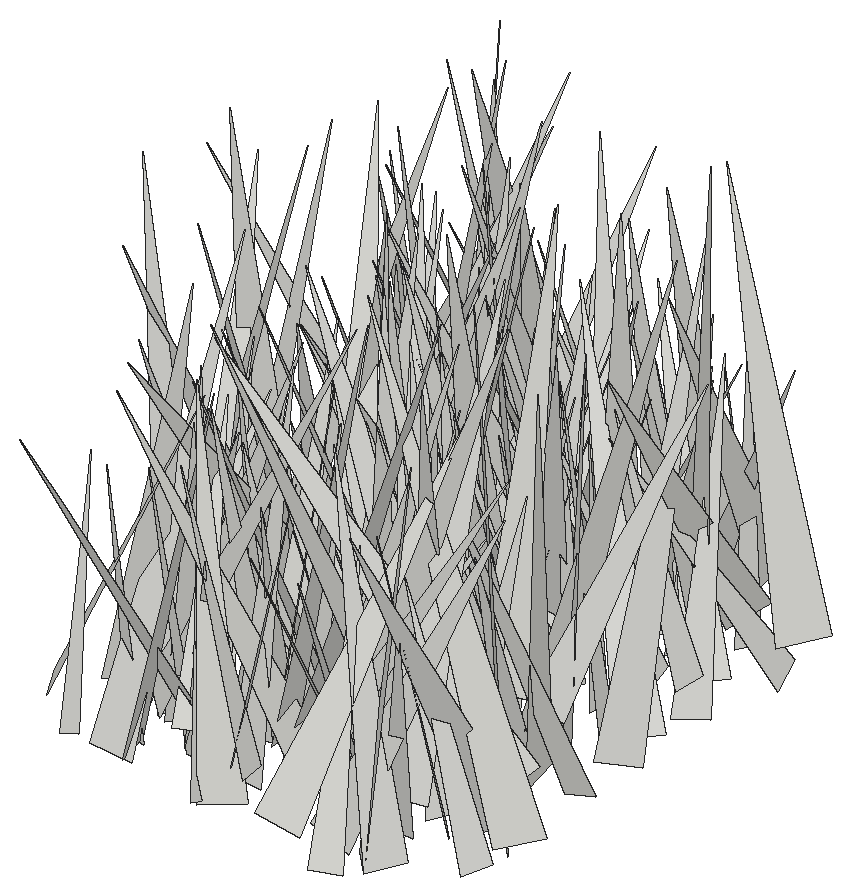
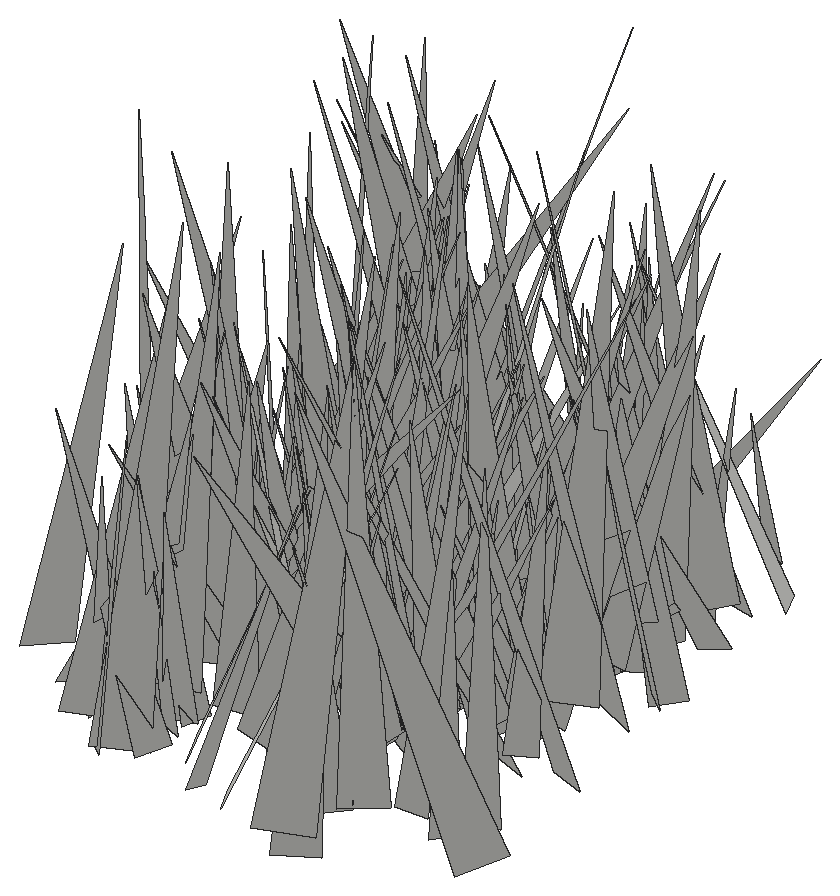
# SketchUp Ruby script. Lengths in inches.
U = 1.inch
M = Sketchup.active_model
def pt(a) = Geom::Point3d.new(a.map { |v| v * U })
def face(e, loops, mat)
  f = e.add_face(loops[0].map { |a| pt(a) })
  loops[1..].each { |l| e.add_face(l.map { |a| pt(a) }).erase! }
  f.material = f.back_material = mat if mat
  f
end
# faces: each face lists its corners as indices into pts; further lists are holes
def faces(e, pts, list, mat = nil) = list.each { |f| face(e, (f[0].is_a?(Array) ? f : [f]).map { |l| l.map { |i| pts[i] } }, mat) }
# xy, xz, yz: faces in a plane at the given z, y or x. An outline is a flat list of corners, or four numbers for a rectangle; further outlines are holes
def ring(l) = l.size == 4 ? [[l[0], l[1]], [l[2], l[1]], [l[2], l[3]], [l[0], l[3]]] : l.each_slice(2).to_a
def flat(e, list, mat, &to3) = list.each { |f| face(e, (f[0].is_a?(Array) ? f : [f]).map { |l| ring(l).map { |u, v| to3.(u, v) } }, mat) }
def xy(e, z, list, mat = nil) = flat(e, list, mat) { |x, y| [x, y, z] }
def xz(e, y, list, mat = nil) = flat(e, list, mat) { |x, z| [x, y, z] }
def yz(e, x, list, mat = nil) = flat(e, list, mat) { |y, z| [x, y, z] }
def lines(e, pts, list) = list.each { |a, b| e.add_line(pt(pts[a]), pt(pts[b])) }
# prism: a flat outline (further loops are holes) pulled along v
def prism(e, loops, v, mat = nil)
  f = face(e, loops, mat); d = Geom::Vector3d.new(v.map { |x| x * U })
  f.pushpull(f.normal.samedirection?(d) ? d.length : -d.length)
end
def box(e, o, s, mat = nil) = prism(e, [[o, [o[0] + s[0], o[1], o[2]], [o[0] + s[0], o[1] + s[1], o[2]], [o[0], o[1] + s[1], o[2]]]], [0, 0, s[2]], mat)
def at(x, y, z, deg = 0) = Geom::Transformation.translation(pt([x, y, z])) * Geom::Transformation.rotation(ORIGIN, Z_AXIS, deg.degrees)
def axes(o, x, y, z) = Geom::Transformation.new([*x, 0, *y, 0, *z, 0, *pt(o).to_a, 1])
def part(name) = M.definitions.add(name)
# library, detail: a bought-in or finely detailed component or shape, given as its bounding box
def library(name, o, s) = part(name).tap { |d| box(d.entities, o, s) }
def detail(e, o, s) = box(e.add_group.entities, o, s)
def put(e, d, t, mat = nil) = e.add_instance(d, t).tap { |i| i.material = mat if mat }
def group(e, t, mat = nil) = e.add_group.tap { |g| g.transformation = t; g.material = mat if mat }.entities
root = M.entities
c1 = part("fur_instance\#9")
p = [[0.8125,0,1.79],[0.67,-0.02,1.48],[0,-0.11,0],[0,0.11,0]]
faces(c1.entities,p,[[0,1,2,3]])
put(root,c1,axes([122.5,103.28,-28.22],[2.81621,-4.35059,0.38195],[-4.36621,-2.81499,0.12899],[-0.09891,0.39082,5.18093]))
put(root,c1,axes([125.08,92.21,-28.22],[-7.4138,3.10521,1.79195],[3.13289,7.61249,-0.22981],[1.74312,-0.47482,8.03455]))
put(root,c1,axes([122.99,104.25,-28.22],[4.3252,-1.84495,1.08949],[-1.74272,-4.45705,-0.62914],[-1.2465,-0.1704,4.65998]))
put(root,c1,axes([124.71,87.48,-27.1],[0.6459,3.9486,0.07217],[3.68247,-0.62859,1.43463],[-1.42692,0.16515,3.73504]))
put(root,c1,axes([122.98,100.89,-27.1],[2.32528,-3.90872,0.2043],[-3.90658,-2.33236,-0.15975],[-0.24182,0.09371,4.54527]))
put(root,c1,axes([123.83,97.73,-27.1],[3.74176,-6.61768,2.63887],[-6.89022,-4.11933,-0.5604],[-1.81167,1.99888,7.58159]))
put(root,c1,axes([124.63,93.51,-28.22],[-3.64093,6.72533,0.73654],[6.73348,3.68347,-0.34805],[0.65778,-0.48058,7.63972]))
put(root,c1,axes([124.44,95.17,-27.1],[0.3349,-5.08877,0.86463],[-5.08924,-0.4702,-0.79617],[-0.86188,0.79915,5.03725]))
put(root,c1,axes([123.36,105.31,-27.1],[-0.67207,-6.04885,0.74296],[-6.03248,0.76649,0.78356],[0.86591,0.6451,6.03542]))
put(root,c1,axes([125.18,97.24,-28.22],[0.28426,-7.43419,0.75555],[-7.30944,-0.43371,-1.51752],[-1.55247,0.68085,7.28321]))
put(root,c1,axes([123.59,95.97,-28.22],[2.95959,7.19025,1.54721],[7.29869,-3.07695,0.338],[-0.90704,-1.29822,7.76818]))
put(root,c1,axes([121.16,104.88,-28.22],[5.54301,-4.89223,1.08245],[-4.92161,-5.01325,2.54471],[0.93987,2.60075,6.94141]))
put(root,c1,axes([121.99,96.09,-27.1],[6.05057,5.41917,1.99571],[5.77348,-5.74186,-1.9125],[-0.1309,-2.76104,7.89425]))
put(root,c1,axes([122.3,99.67,-28.22],[4.03025,7.20792,1.49357],[7.34455,-3.82368,-1.36555],[0.49235,-1.96292,8.14446]))
put(root,c1,axes([126.06,100.875,-27.1],[-4.18794,0.93567,0.33129],[0.9893,4.05153,1.06324],[0.08071,-1.11073,4.15738]))
put(root,c1,axes([125.14,89.89,-28.22],[-1.82115,-3.36265,1.61921],[-3.73204,1.65736,-0.7556],[0.03439,1.7865,3.74875]))
put(root,c1,axes([127.07,101.125,-27.1],[-7.35388,-1.92649,0.06127],[-1.88282,7.23164,1.39751],[0.41243,-1.33667,7.47248]))
put(root,c1,axes([124.92,93.42,-28.22],[-4.28711,2.60894,1.39768],[2.40918,4.50508,-1.01958],[1.71929,0.19268,4.91389]))
put(root,c1,axes([122.51,89.43,-27.1],[4.96423,2.67259,0.04648],[2.6631,-4.93667,-0.5706],[0.22978,-0.52435,5.60898]))
put(root,c1,axes([123.82,91.16,-28.22],[-0.74484,5.04348,0.31723],[4.84937,0.80355,-1.38926],[1.42161,-0.09859,4.90524]))
put(root,c1,axes([127.97,90.31,-28.22],[-2.43401,-4.94438,0.27236],[-4.40728,2.02468,-2.63096],[-2.25763,1.37813,4.84245]))
put(root,c1,axes([122.875,94.39,-28.22],[2.55159,-4.81811,0.15811],[-4.66384,-2.42197,1.46026],[1.21971,0.81832,5.25284]))
put(root,c1,axes([125.04,88.91,-28.22],[1.15921,7.66569,0.40932],[7.66684,-1.17697,0.3294],[-0.3873,-0.35503,7.74584]))
put(root,c1,axes([124.57,105.9375,-27.1],[4.01557,-5.25956,2.05629],[-5.53772,-4.16187,0.169],[-1.10676,1.74125,6.61508]))
put(root,c1,axes([124.03,90.97,-27.1],[5.12868,-4.19399,1.94705],[-4.5125,-5.17419,0.74098],[-1.00889,1.82269,6.58361]))
put(root,c1,axes([124.64,99.09,-27.1],[3.47774,-1.50181,0.39234],[-1.2719,-3.30895,-1.39185],[-0.88975,-1.13996,3.5232]))
put(root,c1,axes([124.42,98.15,-28.22],[3.9235,0.14114,0.37721],[0.06723,-3.8717,0.74932],[-0.3971,0.73898,3.85386]))
put(root,c1,axes([127.51,95.6,-28.22],[-3.53449,-6.31522,1.62159],[-6.50822,3.306,-1.31053],[-0.39309,2.04757,7.11738]))
put(root,c1,axes([124.58,102.7,-28.22],[4.94057,6.27292,2.28459],[6.62263,-4.9638,-0.69253],[-0.84236,-2.23369,7.95482]))
put(root,c1,axes([126.96,101.19,-28.22],[-2.82637,-5.01502,0.69558],[-5.06125,2.81969,-0.23605],[0.13409,0.7222,5.75179]))
put(root,c1,axes([124.77,105.6875,-27.1],[4.05285,-0.43746,0.41546],[-0.3233,-3.95717,-1.01285],[-0.50937,-0.96903,3.94856]))
put(root,c1,axes([124.27,99.93,-28.22],[3.274,7.7332,0.0389],[7.72076,-3.26624,-0.49451],[0.44025,-0.22856,8.38313]))
put(root,c1,axes([126.52,100.1875,-27.1],[-2.91757,4.706,0.99504],[4.75363,2.9987,-0.24403],[0.73452,-0.71423,5.53165]))
put(root,c1,axes([127.03,90.125,-28.22],[-1.86227,-3.58892,1.59018],[-3.91628,1.57852,-1.02377],[-0.26793,1.87217,3.91156]))
put(root,c1,axes([124.77,92.31,-27.1],[4.76351,-2.22786,1.63166],[-2.67424,-4.53288,1.61806],[-0.68857,2.19233,5.00362]))
put(root,c1,axes([125.45,98.64,-28.22],[6.28963,-0.96384,2.1084],[-1.07131,-6.61487,0.17192],[-2.05588,0.49827,6.36073]))
put(root,c1,axes([126.16,97.22,-27.1],[6.60243,-3.6292,1.16999],[-2.40466,-5.77841,-4.35427],[-2.95933,-3.40161,6.14845]))
put(root,c1,axes([127.39,96.2,-28.22],[-5.56313,6.05819,1.00831],[6.02083,5.64819,-0.71719],[1.2116,-0.25113,8.19364]))
put(root,c1,axes([125.4375,108.43,-27.1],[4.78768,-6.87101,0.53821],[-6.76798,-4.81092,-1.21319],[-1.30189,-0.25808,8.28619]))
put(root,c1,axes([127.04,93.37,-28.22],[-5.00491,-0.78513,1.46412],[-0.94309,5.16869,-0.45214],[1.36772,0.69095,5.0459]))
put(root,c1,axes([127.14,102.01,-27.1],[5.31118,5.11176,2.74997],[4.78098,-5.96627,1.85658],[-3.29161,-0.41778,7.13385]))
put(root,c1,axes([125.53,91.66,-28.22],[4.04014,-3.74392,1.13553],[-3.80741,-4.13804,-0.09691],[-0.90002,0.69913,5.50729]))
put(root,c1,axes([128.55,99.65,-28.22],[-7.00273,-0.39667,0.95685],[-0.59042,6.90153,-1.45992],[0.85107,1.52402,6.86034]))
put(root,c1,axes([127.22,98.15,-28.22],[-3.60239,-0.15597,0.87969],[-0.19043,3.7046,-0.12301],[0.87288,0.16452,3.60367]))
put(root,c1,axes([125.39,89.45,-28.22],[5.7925,1.49056,1.34896],[1.52882,-5.93778,-0.00376],[-1.30544,-0.3399,5.9812]))
put(root,c1,axes([127.21,89.71,-27.1],[-2.44616,4.11048,0.29857],[4.09909,2.46258,-0.31948],[0.42742,-0.0923,4.7726]))
put(root,c1,axes([125.58,107.7,-28.22],[4.30968,-5.09044,0.61484],[-5.06109,-4.35201,-0.55619],[-0.82219,0.10671,6.64655]))
put(root,c1,axes([127.07,94.18,-27.1],[1.11597,-3.30458,1.27259],[-3.40234,-1.37051,-0.57526],[-0.98175,0.99326,3.44016]))
put(root,c1,axes([127.21,93.55,-28.22],[-4.48164,3.41054,1.04148],[3.17852,4.57879,-1.31654],[1.61662,0.45221,5.47573]))
put(root,c1,axes([129.2,103.3,-27.1],[-7.32876,-0.97242,0.83606],[-1.07916,7.29688,-0.97277],[0.69283,1.07947,7.32872]))
put(root,c1,axes([125.67,95.92,-28.22],[4.93042,2.67254,1.54888],[2.99605,-4.84755,-1.1728],[-0.75178,-1.79146,5.48417]))
put(root,c1,axes([128.22,104.02,-28.22],[-4.66446,-0.17714,0.77084],[-0.14932,4.72517,0.1823],[0.77671,-0.15541,4.66426]))
put(root,c1,axes([124.67,100.06,-27.1],[6.16079,-1.33707,0.34037],[-1.37023,-6.11166,0.79308],[-0.16154,0.84778,6.25413]))
put(root,c1,axes([127.18,97.35,-27.1],[-2.4025,-2.92839,0.44923],[-2.80853,2.4353,0.85486],[0.94311,-0.20767,3.69008]))
put(root,c1,axes([128.77,88.4,-28.22],[-6.05954,0.33778,0.89505],[0.02694,5.79744,-2.00555],[0.95629,1.97708,5.728]))
put(root,c1,axes([128.68,100.66,-27.1],[0.56796,-5.36738,0.34113],[-5.01782,-0.65229,-1.90884],[-1.93561,0.11605,5.04853]))
put(root,c1,axes([129.16,106.4375,-28.22],[-5.15654,-2.89646,0.02201],[-2.88562,5.14083,0.47427],[0.2514,-0.40276,5.89529]))
put(root,c1,axes([128.62,101.76,-27.1],[1.86893,4.92203,0.04113],[4.36091,-1.67616,2.42774],[-2.28266,0.8277,4.67176]))
put(root,c1,axes([126.3125,105.0625,-28.22],[3.18493,-3.37138,0.77047],[-3.44968,-3.17103,0.3845],[-0.24394,0.82581,4.62191]))
put(root,c1,axes([126.41,102.44,-27.1],[5.41159,0.09186,1.28906],[0.07062,-5.56242,0.09991],[-1.29039,0.08081,5.41145]))
put(root,c1,axes([127.11,102.1,-27.1],[-1.46748,5.77462,2.34569],[6.13429,1.76496,-0.50731],[1.10405,-2.13089,5.93652]))
put(root,c1,axes([127.42,100.625,-27.1],[0.8568,-5.86099,0.80486],[-5.91149,-0.87995,-0.11477],[-0.231,0.77949,5.92218]))
put(root,c1,axes([128.22,105.14,-27.1],[-3.59271,-3.52154,0.36411],[-3.38524,3.56898,1.11534],[1.03633,-0.55007,4.90559]))
put(root,c1,axes([128.3,92.16,-28.22],[0.40641,-5.35004,1.66525],[-5.54368,-0.62666,-0.66032],[-0.81458,1.59547,5.32467]))
put(root,c1,axes([126.89,90.57,-28.22],[2.03296,-3.43324,0.36978],[-3.45285,-2.01606,0.26469],[0.04074,0.45292,3.9812]))
put(root,c1,axes([127.39,91.125,-28.22],[2.94995,3.39967,1.09614],[3.50655,-3.02709,-0.04841],[-0.68072,-0.86052,4.50085]))
put(root,c1,axes([129.93,95.78,-28.22],[-5.4054,2.23783,0.44972],[2.26041,5.40869,0.2551],[0.31726,-0.40826,5.84475]))
put(root,c1,axes([129.29,104.84,-27.1],[-0.74587,-6.40704,1.23448],[-6.45249,0.53969,-1.09751],[-0.96927,1.33753,6.35625]))
put(root,c1,axes([127.55,101,-28.22],[-5.17652,4.83446,1.05401],[3.91261,4.93311,-3.41105],[3.02894,1.88989,6.20751]))
put(root,c1,axes([130.46,92.89,-28.22],[-2.94744,-5.34651,0.76174],[-5.29498,2.69026,-1.60576],[-1.06233,1.42484,5.89017]))
put(root,c1,axes([126.07,99.46,-27.1],[3.27115,-5.93629,2.22387],[-6.24966,-2.60094,2.25],[1.06155,2.98013,6.39355]))
put(root,c1,axes([130.375,91.33,-28.22],[-6.87561,-0.89332,0.66489],[-0.69538,6.69239,1.80069],[0.86979,-1.71115,6.69549]))
put(root,c1,axes([129.24,88.57,-28.22],[-3.57367,4.96866,1.72232],[5.21894,3.60663,0.42422],[0.64547,-1.65218,6.10563]))
put(root,c1,axes([125.23,90.57,-27.1],[5.08074,5.57509,0.64514],[5.46993,-4.72427,-2.25231],[1.25607,-1.97773,7.19879]))
put(root,c1,axes([131.49,93.66,-28.22],[-5.18196,-4.15409,0.26027],[-4.02731,4.89921,-1.98883],[-1.05116,1.70828,6.3367]))
put(root,c1,axes([129.84,98.58,-28.22],[-7.87878,-1.52664,2.20407],[-1.70967,8.13085,-0.47967],[2.06533,0.90687,8.01097]))
put(root,c1,axes([128.19,92.67,-28.22],[4.42301,-0.66017,1.25029],[-0.31732,-4.46498,-1.23502],[-1.37781,-1.09094,4.29808]))
put(root,c1,axes([130.38,97.59,-27.1],[-4.86082,-0.82699,0.28427],[-0.77768,4.82218,0.73078],[0.39992,-0.67448,4.87621]))
put(root,c1,axes([130.04,88.875,-27.1],[-4.57594,-0.69447,0.70937],[-0.73517,4.61906,-0.2203],[0.6671,0.32667,4.62309]))
put(root,c1,axes([130.01,94.16,-27.1],[1.21236,6.8418,0.01969],[6.58716,-1.17263,1.87473],[-1.84929,0.30844,6.6907]))
put(root,c1,axes([128.9375,89.93,-28.22],[1.06492,5.99669,1.55027],[6.17359,-1.15473,0.22589],[-0.50038,-1.48458,6.08632]))
put(root,c1,axes([129.68,96.99,-28.22],[-5.57338,-5.53642,0.81265],[-5.27737,5.58191,1.83481],[1.86058,-0.75178,7.63858]))
put(root,c1,axes([128.1,98.21,-27.1],[7.25129,-2.23194,2.73946],[-2.93898,-7.28136,1.84704],[-1.96177,2.6585,7.35875]))
put(root,c1,axes([134.1875,100.6,-27.1],[-5.38862,-5.55187,0.24968],[-4.68183,4.34761,-4.37054],[-2.99434,3.19341,6.38427]))
put(root,c1,axes([130.23,106.39,-28.22],[-4.47409,-0.55232,0.95951],[-0.288,4.43762,1.21151],[1.069,-1.11608,4.34221]))
put(root,c1,axes([129.16,94.58,-28.22],[5.828,-3.21448,3.45143],[-4.0564,-6.21538,1.06086],[-2.40642,2.69201,6.57061]))
put(root,c1,axes([130.8,94.84,-28.22],[5.10712,-2.96498,5.20518],[-4.57955,-6.3419,0.88079],[-3.86171,3.59957,5.83935]))
put(root,c1,axes([131.67,104.77,-28.22],[-5.05494,-2.22544,0.30278],[-2.23904,4.935,-1.10864],[-0.17591,1.1357,5.41072]))
put(root,c1,axes([131.78,99.42,-27.1],[-4.01783,2.35497,0.3103],[2.27352,3.63609,1.84258],[-0.68795,-1.73727,4.27712]))
put(root,c1,axes([130.64,98.13,-27.1],[-5.01766,-1.40088,1.70753],[-1.93126,4.83928,-1.7049],[1.07162,2.16194,4.92267]))
put(root,c1,axes([129.11,92.55,-27.1],[-3.54773,2.23846,2.32232],[2.39169,4.14191,-0.33862],[2.16418,-0.90784,4.1812]))
put(root,c1,axes([130.97,102,-27.1],[-7.04471,-1.4589,1.32068],[-0.96261,6.83613,2.41686],[1.71638,-2.15394,6.77607]))
put(root,c1,axes([130.78,103.87,-27.1],[-2.14866,5.91991,1.32548],[6.06222,2.04254,0.70466],[-0.22751,-1.48381,6.25824]))
put(root,c1,axes([129.02,101.34,-27.1],[3.30079,2.00098,0.99665],[2.11543,-3.37049,-0.23912],[-0.72261,-0.72685,3.85253]))
put(root,c1,axes([129.34,100.34,-27.1],[2.40943,-6.40182,1.38295],[-6.51779,-2.4885,-0.16399],[-0.64358,1.23501,6.83826]))
put(root,c1,axes([129.16,89.17,-27.1],[-3.23487,-1.73884,2.61208],[-2.22596,3.91581,-0.14997],[2.2117,1.39779,3.66954]))
put(root,c1,axes([132.13,94.79,-27.1],[-5.92654,3.46188,1.28835],[3.68281,5.72588,1.55549],[0.28525,-1.99951,6.68498]))
put(root,c1,axes([130.74,99.92,-27.1],[3.92843,5.06138,3.38638],[5.5366,-4.64662,0.52215],[-2.53598,-2.30413,6.38572]))
put(root,c1,axes([130.04,101.38,-28.22],[-3.2792,-1.26365,1.37089],[-0.97388,3.52607,0.9207],[1.58988,-0.44645,3.3915]))
put(root,c1,axes([133.17,98.52,-28.22],[-4.03956,-5.75099,0.92293],[-5.66396,3.6166,-2.25467],[-1.3584,2.0224,6.65646]))
put(root,c1,axes([129.85,96.04,-27.1],[-4.92901,3.2655,3.81824],[4.17297,5.6397,0.56365],[2.798,-2.65855,5.88565]))
put(root,c1,axes([129.49,91.01,-27.1],[6.35559,1.23086,1.81432],[1.1106,-6.60444,0.5901],[-1.89033,0.25813,6.44673]))
put(root,c1,axes([131.25,99.02,-28.22],[4.80769,-4.80499,2.60276],[-4.52111,-5.44469,-1.70033],[-3.0695,0.49361,6.58109]))
put(root,c1,axes([130.94,99.37,-28.22],[-5.21619,-2.22313,1.39253],[-1.54183,5.10575,2.37575],[2.12232,-1.75473,5.14847]))
put(root,c1,axes([130.77,94.09,-27.1],[4.6761,-4.10232,2.76945],[-4.45315,-5.14998,-0.1096],[-2.16064,1.73593,6.21956]))
put(root,c1,axes([131.96,97.45,-28.22],[0.51601,7.02264,0.2402],[6.84431,-0.55684,1.57697],[-1.5908,-0.11784,6.86272]))
put(root,c1,axes([131.39,99.12,-27.1],[2.56304,5.03632,1.18387],[4.82189,-2.80423,1.49027],[-1.87495,-0.32715,5.45094]))
put(root,c1,axes([132.99,94.48,-28.22],[-5.13567,3.95215,0.39173],[3.97037,5.09374,0.66187],[-0.09557,-0.76314,6.44644]))
put(root,c1,axes([132.01,101.33,-27.1],[-1.08629,-5.09453,1.21583],[-5.17343,0.84989,-1.06105],[-0.81738,1.39139,5.09985]))
put(root,c1,axes([128.05,103.58,-27.1],[5.66121,2.03663,0.41958],[1.99596,-4.98096,-2.75306],[0.58316,-2.72311,5.34956]))
put(root,c1,axes([132.32,91.59,-27.1],[-7.61718,0.0241,1.98426],[-0.51537,7.57673,-2.07045],[1.91631,2.1335,7.33043]))
put(root,c1,axes([131.86,96.45,-27.1],[-3.13424,-4.33981,2.11732],[-4.81159,3.01955,-0.93345],[0.40688,2.2779,5.27125]))
put(root,c1,axes([130.07,102.09,-28.22],[2.49567,-4.97649,0.70111],[-5.02561,-2.47346,0.33254],[-0.01412,0.77585,5.55727]))
put(root,c1,axes([131.35,100.02,-27.1],[-4.05743,3.11883,1.27429],[2.94276,4.25195,-1.03673],[1.64046,0.08657,5.0115]))
put(root,c1,axes([132.49,92.68,-27.1],[-7.22673,-3.69522,1.05519],[-3.3656,7.17065,2.06111],[1.85494,-1.38592,7.85061]))
put(root,c1,axes([131.42,96.62,-27.1],[-4.23654,2.45749,2.21286],[2.8358,4.54981,0.37637],[1.70124,-1.46429,4.88322]))
put(root,c1,axes([130.4,99.95,-28.22],[4.75922,3.00167,0.77273],[2.8511,-4.79497,1.06623],[-1.21588,0.50555,5.5248]))
put(root,c1,axes([131.25,99.39,-27.1],[-3.49002,4.97532,0.38419],[4.70613,3.43753,-1.76559],[1.65943,0.71499,5.81522]))
put(root,c1,axes([132.03,90.87,-27.1],[-2.1706,-3.79382,0.07549],[-3.76138,2.16267,0.53397],[0.50075,-0.20018,4.33814]))
put(root,c1,axes([133,94.99,-28.22],[-5.2528,1.04607,1.18822],[1.28573,5.22141,1.0871],[0.92359,-1.31932,5.24446]))
put(root,c1,axes([129.28,91.875,-28.22],[8.28106,0.30024,0.90595],[0.31898,-8.32832,-0.15571],[-0.89952,-0.18935,8.28504]))
put(root,c1,axes([131.42,98.03,-28.22],[2.50571,3.8301,0.73521],[3.84486,-2.57244,0.29737],[-0.65369,-0.44905,4.56726]))
put(root,c1,axes([132.65,92.72,-28.22],[-3.74669,3.50171,1.17991],[3.59906,3.83892,0.03541],[0.8372,-0.8322,5.12819]))
put(root,c1,axes([130.07,93.15,-27.1],[0.48143,3.7055,0.846],[3.27794,0.02687,-1.98307],[1.92393,-0.97302,3.16701]))
put(root,c1,axes([133.84,98.37,-27.1],[-4.92435,-0.05312,0.24709],[-0.15186,4.47527,-2.06445],[0.20202,2.06935,4.47102]))
put(root,c1,axes([133.05,95.73,-27.1],[0.28684,-3.45624,1.82339],[-3.70035,-0.82791,-0.9872],[-1.25608,1.64973,3.32465]))
put(root,c1,axes([133.53,94.92,-28.22],[-5.37487,-0.5228,0.79074],[-0.44432,5.41107,0.55741],[0.83736,-0.48456,5.37139]))
put(root,c1,axes([129.73,103,-28.22],[6.9866,-0.46387,0.39437],[-0.38095,-6.874,-1.33651],[-0.47495,-1.31005,6.87325]))
put(root,c1,axes([132.93,103.69,-28.22],[-1.86481,4.13252,0.34952],[4.14724,1.85655,0.17621],[-0.01744,-0.39104,4.53037]))
put(root,c1,axes([132.23,91.1875,-28.22],[-1.29347,-4.18784,0.40951],[-4.17089,1.33267,0.45438],[0.55623,0.25449,4.35943]))
put(root,c1,axes([131.96,97.49,-27.1],[4.64418,-2.47093,1.08294],[-2.19439,-4.71399,-1.3452],[-1.56935,-0.72073,5.0857]))
put(root,c1,axes([136.13,92.87,-27.1],[-7.44265,2.94787,0.75024],[2.95668,6.54484,3.6151],[-0.71474,-3.62229,7.14241]))
put(root,c1,axes([130.67,91.76,-27.1],[2.74298,6.25055,1.8619],[6.47418,-2.36552,-1.59662],[0.78801,-2.32269,6.63657]))
put(root,c1,axes([132.88,89.92,-28.22],[3.09687,5.17866,0.3937],[4.90573,-3.06729,1.75775],[-1.70508,0.58082,5.7723]))
put(root,c1,axes([134.18,101.75,-28.22],[-4.25232,-1.15186,0.17503],[-1.13335,4.24309,0.38907],[0.27009,-0.33025,4.38835]))
put(root,c1,axes([132.7,96.68,-27.1],[-2.30774,6.81626,2.09214],[7.04491,2.51871,-0.43516],[1.09893,-1.8327,7.18315]))
put(root,c1,axes([131.31,100.29,-27.1],[2.32461,-5.72045,0.33614],[-5.68592,-2.25756,0.90225],[0.71192,0.64824,6.10846]))
put(root,c1,axes([132.98,103.82,-27.1],[2.11565,-6.08651,1.80009],[-6.2822,-2.27872,-0.32139],[-0.90548,1.58863,6.43571]))
put(root,c1,axes([134.06,95.24,-27.1],[0.22156,-4.52657,1.23949],[-4.53883,-0.5223,-1.09609],[-1.19379,1.1457,4.39744]))
put(root,c1,axes([132.81,104.29,-28.22],[1.65832,3.59632,1.35209],[3.82471,-1.68517,-0.20869],[-0.36513,-1.31848,3.95475]))
put(root,c1,axes([134.53,92.01,-28.22],[-6.31107,2.62453,1.38258],[2.63294,6.45317,-0.23139],[1.36651,-0.31261,6.83112]))
put(root,c1,axes([132.96,89.625,-28.22],[-2.34168,-2.41248,1.9117],[-2.76899,2.70012,0.01564],[1.3444,1.35921,3.36204]))
put(root,c1,axes([133.85,102.99,-28.22],[-4.57761,1.25738,1.06742],[0.91701,4.55759,-1.43608],[1.37093,1.14988,4.52473]))
put(root,c1,axes([131.77,101.19,-28.22],[4.92859,0.75105,0.39032],[0.57555,-4.66461,1.7081],[-0.62062,1.63853,4.68375]))
put(root,c1,axes([134.01,99.25,-28.22],[-3.8319,-0.08961,1.0116],[-0.27638,3.8917,-0.7022],[0.97723,0.7493,3.76807]))
put(root,c1,axes([133.875,87.33,-28.22],[-1.31854,4.49628,0.43937],[4.51767,1.31381,0.11263],[0.01505,-0.45333,4.68427]))
put(root,c1,axes([133.88,103.55,-27.1],[1.42768,-3.34431,1.65268],[-3.54003,-1.77266,-0.52903],[-1.17641,1.27565,3.59761]))
put(root,c1,axes([132.59,101.93,-27.1],[2.16747,-6.96935,1.82134],[-7.20329,-2.08612,0.58967],[0.04123,1.91397,7.27476]))
put(root,c1,axes([133.24,106,-28.22],[4.41778,-6.32124,1.65754],[-6.32459,-4.6393,-0.83587],[-1.6447,0.86086,7.66656]))
put(root,c1,axes([132.91,91.84,-27.1],[7.20277,3.49638,1.97973],[3.12762,-7.42996,1.74287],[-2.5223,0.77133,7.81454]))
put(root,c1,axes([135.37,102.35,-28.22],[-3.54308,4.52564,0.44169],[4.5332,3.47169,0.79207],[-0.35583,-0.83417,5.69276]))
put(root,c1,axes([135.03,88.55,-28.22],[-5.60882,2.54428,1.1021],[2.59069,5.69507,0.03704],[0.9881,-0.48955,6.15881]))
put(root,c1,axes([135.89,98.7,-28.22],[-3.78417,5.30239,0.2634],[5.25954,3.70033,1.07214],[-0.72248,-0.83479,6.42541]))
put(root,c1,axes([132.09,100.09,-27.1],[4.65437,1.55789,0.49043],[1.62302,-4.57734,-0.86283],[-0.1826,-0.97553,4.83174]))
put(root,c1,axes([132.41,87.04,-27.1],[-1.13308,6.40977,0.66119],[6.08836,1.28481,-2.02171],[2.11049,-0.26515,6.18722]))
put(root,c1,axes([132.5625,103.44,-28.22],[4.88822,-0.89007,0.63341],[-0.87396,-4.92864,-0.18113],[-0.65546,-0.06625,4.96529]))
put(root,c1,axes([133.44,94.46,-27.1],[-1.54021,3.23682,1.39983],[3.28512,1.87235,-0.71486],[1.28237,-0.90889,3.51258]))
put(root,c1,axes([132.5,94.03,-28.22],[0.39282,-7.92697,1.06347],[-7.86049,-0.18606,1.51663],[1.47665,1.11832,7.79044]))
put(root,c1,axes([133.74,106.44,-28.22],[-2.90046,-3.39812,1.38689],[-3.27993,3.19309,0.96417],[1.64705,0.37459,4.36237]))
put(root,c1,axes([135.13,102.39,-27.1],[-4.98874,-1.77944,1.14235],[-1.81158,5.1064,0.04294],[1.09068,0.3424,5.29642]))
put(root,c1,axes([135.9,97.35,-28.22],[-5.16392,-1.1559,0.80889],[-1.35151,4.93357,-1.57791],[0.40477,1.72635,5.05098]))
put(root,c1,axes([131.92,90.43,-27.1],[6.06814,-4.77445,2.10475],[-5.2154,-5.64781,2.22478],[-0.15808,3.05854,7.39379]))
put(root,c1,axes([135.04,104.54,-28.22],[-4.45117,0.87592,1.04433],[0.68712,4.52233,-0.86441],[1.17717,0.67238,4.45342]))
put(root,c1,axes([132.43,105.53,-28.22],[4.45339,-2.56263,0.11815],[-2.55046,-4.39735,0.75645],[0.27609,0.71411,5.08208]))
put(root,c1,axes([134.07,90.27,-27.1],[-2.77927,7.20298,1.80131],[7.21654,3.07297,-1.15349],[1.74623,-1.2353,7.63392]))
put(root,c1,axes([134.31,88.4,-28.22],[-3.91577,-3.49387,3.17429],[-4.26524,4.38586,-0.43413],[2.02262,2.48468,5.2299]))
put(root,c1,axes([134.49,97.24,-28.22],[3.82157,4.19761,2.25189],[4.45533,-4.17126,0.21447],[-1.68552,-1.50865,5.67259]))
put(root,c1,axes([131.36,89.625,-27.1],[4.19059,5.13354,0.34706],[4.85008,-3.79176,-2.47669],[1.71767,-1.81771,6.14657]))
put(root,c1,axes([134.22,95.4,-28.22],[3.93846,-2.19121,0.70559],[-1.95473,-3.92185,-1.26841],[-1.21585,-0.79274,4.32481]))
put(root,c1,axes([134.24,106.72,-27.1],[6.25747,-1.85529,1.59771],[-1.00282,-5.94215,-2.97253],[-2.23363,-2.52972,5.81052]))
put(root,c1,axes([138.32,90.37,-27.1],[-2.68904,7.46116,1.26428],[7.06219,1.99214,3.26422],[-2.71897,-2.20471,7.22805]))
put(root,c1,axes([134,90.36,-28.22],[0.84886,-4.32385,0.54485],[-4.30912,-0.7498,0.76315],[0.65118,0.6747,4.3398]))
put(root,c1,axes([133.5,97.33,-28.22],[7.44072,-1.6859,2.03296],[-2.09272,-7.4711,1.46382],[-1.61112,1.91833,7.48758]))
put(root,c1,axes([136.64,95.14,-28.22],[-0.6126,-5.21006,0.97224],[-5.10965,0.32064,-1.50131],[-1.40764,1.1035,5.02654]))
put(root,c1,axes([136.32,100.35,-27.1],[-4.20728,0.83557,0.99678],[1.00115,4.23485,0.67581],[0.83033,-0.87227,4.23588]))
put(root,c1,axes([136.28,89.7,-27.1],[-3.38614,-3.10021,1.02366],[-3.22386,3.40798,-0.34286],[0.51569,0.94841,4.57818]))
put(root,c1,axes([136.39,97.14,-28.22],[-6.77077,3.15469,0.89527],[2.64884,6.47215,-2.77341],[1.93319,2.18084,6.93567]))
put(root,c1,axes([132.79,88.87,-28.22],[0.63179,6.0642,2.01169],[5.81387,0.29266,-2.70812],[2.6496,-2.08816,5.46258]))
put(root,c1,axes([136.87,103.94,-28.22],[-5.02387,-1.18033,0.42976],[-0.88594,4.58548,2.23734],[0.8905,-2.09699,4.65046]))
put(root,c1,axes([135.22,104.36,-27.1],[5.40671,-4.03304,0.21931],[-3.53675,-4.90438,-2.9974],[-1.95061,-2.2864,6.04264]))
put(root,c1,axes([134.89,102.49,-27.1],[4.42565,6.01002,3.52258],[6.87552,-4.43985,-1.06317],[-1.12079,-3.50468,7.38759]))
put(root,c1,axes([135.13,95.2,-28.22],[6.36794,0.62079,2.33056],[0.97414,-6.68136,-0.88201],[-2.20634,-1.15823,6.33704]))
put(root,c1,axes([136.36,100.37,-28.22],[-3.96377,3.38106,0.80717],[3.27975,4.04327,-0.83051],[1.15166,0.12228,5.14327]))
put(root,c1,axes([137.33,104.14,-27.1],[-5.93712,3.87569,1.72238],[4.1151,5.9813,0.72589],[1.02637,-1.56207,7.0529]))
put(root,c1,axes([137.07,90.04,-28.22],[-3.9914,1.89648,0.82188],[2.01712,3.964,0.64912],[0.45094,-0.94526,4.3711]))
put(root,c1,axes([136.08,92.46,-28.22],[4.00993,-5.51552,0.33203],[-5.14979,-3.87921,-2.24547],[-2.00271,-1.06842,6.43882]))
put(root,c1,axes([134.17,96.67,-27.1],[-0.28996,5.60424,1.15409],[5.32871,0.68543,-1.98963],[2.08431,-0.97272,5.24719]))
put(root,c1,axes([136.74,91.72,-28.22],[-5.85102,-5.01294,3.05498],[-5.59861,6.06235,-0.77491],[1.76582,2.61061,7.66574]))
